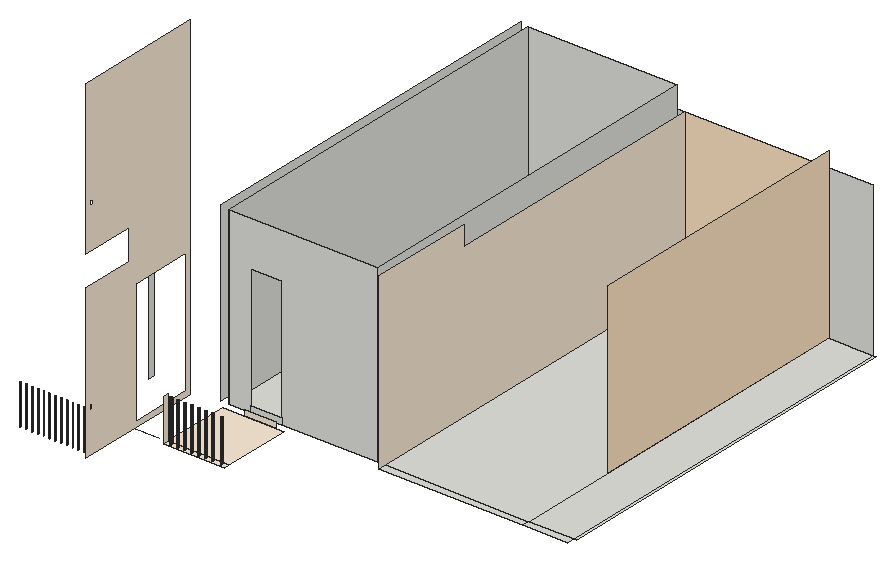
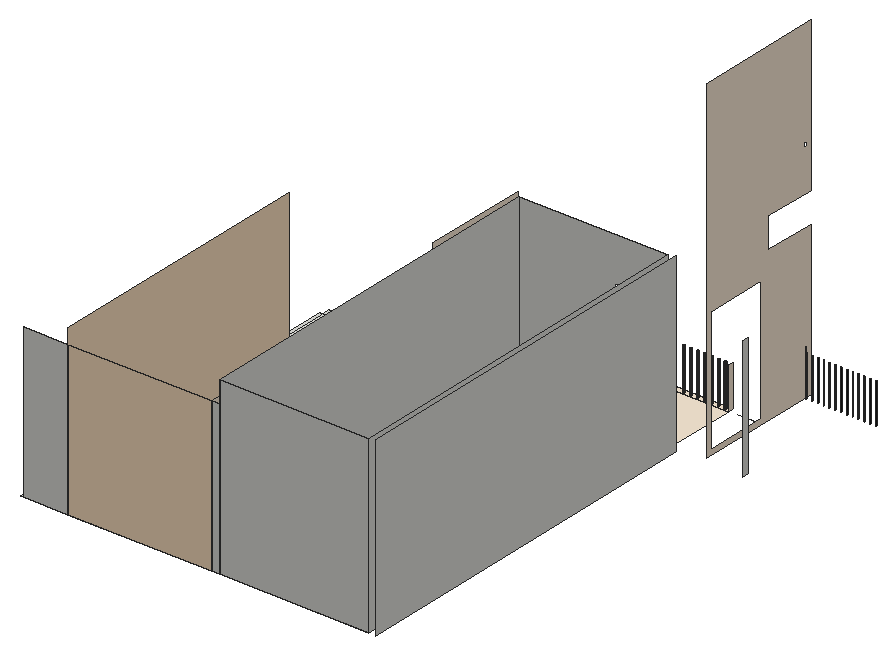
# SketchUp Ruby script. Lengths in inches.
U = 1.inch
M = Sketchup.active_model
def pt(a) = Geom::Point3d.new(a.map { |v| v * U })
def face(e, loops, mat)
  f = e.add_face(loops[0].map { |a| pt(a) })
  loops[1..].each { |l| e.add_face(l.map { |a| pt(a) }).erase! }
  f.material = f.back_material = mat if mat
  f
end
# faces: each face lists its corners as indices into pts; further lists are holes
def faces(e, pts, list, mat = nil) = list.each { |f| face(e, (f[0].is_a?(Array) ? f : [f]).map { |l| l.map { |i| pts[i] } }, mat) }
# xy, xz, yz: faces in a plane at the given z, y or x. An outline is a flat list of corners, or four numbers for a rectangle; further outlines are holes
def ring(l) = l.size == 4 ? [[l[0], l[1]], [l[2], l[1]], [l[2], l[3]], [l[0], l[3]]] : l.each_slice(2).to_a
def flat(e, list, mat, &to3) = list.each { |f| face(e, (f[0].is_a?(Array) ? f : [f]).map { |l| ring(l).map { |u, v| to3.(u, v) } }, mat) }
def xy(e, z, list, mat = nil) = flat(e, list, mat) { |x, y| [x, y, z] }
def xz(e, y, list, mat = nil) = flat(e, list, mat) { |x, z| [x, y, z] }
def yz(e, x, list, mat = nil) = flat(e, list, mat) { |y, z| [x, y, z] }
def lines(e, pts, list) = list.each { |a, b| e.add_line(pt(pts[a]), pt(pts[b])) }
# prism: a flat outline (further loops are holes) pulled along v
def prism(e, loops, v, mat = nil)
  f = face(e, loops, mat); d = Geom::Vector3d.new(v.map { |x| x * U })
  f.pushpull(f.normal.samedirection?(d) ? d.length : -d.length)
end
def box(e, o, s, mat = nil) = prism(e, [[o, [o[0] + s[0], o[1], o[2]], [o[0] + s[0], o[1] + s[1], o[2]], [o[0], o[1] + s[1], o[2]]]], [0, 0, s[2]], mat)
def at(x, y, z, deg = 0) = Geom::Transformation.translation(pt([x, y, z])) * Geom::Transformation.rotation(ORIGIN, Z_AXIS, deg.degrees)
def axes(o, x, y, z) = Geom::Transformation.new([*x, 0, *y, 0, *z, 0, *pt(o).to_a, 1])
def part(name) = M.definitions.add(name)
# library, detail: a bought-in or finely detailed component or shape, given as its bounding box
def library(name, o, s) = part(name).tap { |d| box(d.entities, o, s) }
def detail(e, o, s) = box(e.add_group.entities, o, s)
def put(e, d, t, mat = nil) = e.add_instance(d, t).tap { |i| i.material = mat if mat }
def group(e, t, mat = nil) = e.add_group.tap { |g| g.transformation = t; g.material = mat if mat }.entities
root = M.entities
M.materials.add("[0012_Bisque]").color = [255, 228, 196]
M.materials.add("[0028_AntiqueWhite]").color = [250, 235, 215]
M.materials.add("[Color M08]").color = [30, 30, 30]
xy(root,177,[[355.625,292.4375,468.75,298.4375],[468.75,292.4375,503.75,298.4375],[232.3125,298.4375,349.625,592.9375],[355.625,298.4375,468.75,592.9375],[468.75,298.4375,503.75,592.9375],
  [503.75,298.4375,506.4375,592.9375]])
xy(root,177,[[[232.3125,234.5,280.54,238.33],[242.01,235.93,241.83,235.95,241.66,236.02,241.52,236.12,241.41,236.26,241.34,236.43,241.31,236.61,241.33,236.78,241.39,236.95,241.5,237.09,241.64,237.21,241.81,237.28,241.98,237.31,242.16,237.29,242.33,237.22,242.47,237.11,242.58,236.97,242.66,236.81,242.68,236.63,242.66,236.45,242.6,236.29,242.49,236.14,242.35,236.03,242.1875,235.96],[247.45,235.93,247.27,235.95,247.1,236.02,246.96,236.12,246.84,236.26,246.77,236.43,246.75,236.61,246.77,236.78,246.83,236.95,246.9375,237.09,247.08,237.21,247.24,237.28,247.42,237.31,247.6,237.29,247.77,237.22,247.91,237.11,248.02,236.97,248.09,236.81,248.12,236.63,248.1,236.45,248.04,236.29,247.93,236.14,247.79,236.03,247.625,235.96],[252.88,235.93,252.71,235.95,252.54,236.02,252.39,236.12,252.28,236.26,252.21,236.43,252.18,236.61,252.2,236.78,252.27,236.95,252.375,237.09,252.52,237.21,252.68,237.28,252.86,237.31,253.04,237.29,253.2,237.22,253.35,237.11,253.46,236.97,253.53,236.81,253.56,236.63,253.54,236.45,253.47,236.29,253.37,236.14,253.23,236.03,253.0625,235.96],[258.32,235.93,258.14,235.95,257.98,236.02,257.83,236.12,257.72,236.26,257.65,236.43,257.62,236.61,257.64,236.78,257.71,236.95,257.8125,237.09,257.95,237.21,258.12,237.28,258.3,237.31,258.47,237.29,258.64,237.22,258.79,237.11,258.9,236.97,258.97,236.81,259,236.63,258.98,236.45,258.91,236.29,258.8,236.14,258.66,236.03,258.5,235.96],[263.76,235.93,263.58,235.95,263.41,236.02,263.27,236.12,263.16,236.26,263.09,236.43,263.06,236.61,263.08,236.78,263.14,236.95,263.25,237.09,263.39,237.21,263.56,237.28,263.73,237.31,263.91,237.29,264.08,237.22,264.22,237.11,264.33,236.97,264.41,236.81,264.43,236.63,264.41,236.45,264.35,236.29,264.24,236.14,264.1,236.03,263.9375,235.96],[269.26,235.93,269.08,235.95,268.91,236.02,268.77,236.12,268.66,236.26,268.59,236.43,268.56,236.61,268.58,236.78,268.64,236.95,268.75,237.09,268.89,237.21,269.06,237.28,269.23,237.31,269.41,237.29,269.58,237.22,269.72,237.11,269.83,236.97,269.91,236.81,269.93,236.63,269.91,236.45,269.85,236.29,269.74,236.14,269.6,236.03,269.4375,235.96],[276.2,235.93,276.02,235.95,275.85,236.02,275.71,236.12,275.59,236.26,275.52,236.43,275.5,236.61,275.52,236.78,275.58,236.95,275.6875,237.09,275.83,237.21,275.99,237.28,276.17,237.31,276.35,237.29,276.52,237.22,276.66,237.11,276.77,236.97,276.84,236.81,276.87,236.63,276.85,236.45,276.79,236.29,276.68,236.14,276.54,236.03,276.375,235.96],[236.57,235.93,236.39,235.95,236.23,236.02,236.08,236.12,235.97,236.26,235.9,236.43,235.87,236.61,235.89,236.78,235.96,236.95,236.0625,237.09,236.2,237.21,236.37,237.28,236.55,237.31,236.72,237.29,236.89,237.22,237.04,237.11,237.15,236.97,237.22,236.81,237.25,236.63,237.23,236.45,237.16,236.29,237.05,236.14,236.91,236.03,236.75,235.96]],[232.3125,238.33,280.54,292.4375]],"[0028_AntiqueWhite]")
xy(root,177,[[236.57,235.93,236.39,235.95,236.23,236.02,236.08,236.12,235.97,236.26,235.9,236.43,235.87,236.61,235.89,236.78,235.96,236.95,236.0625,237.09,236.2,237.21,236.37,237.28,236.55,237.31,236.72,237.29,236.89,237.22,237.04,237.11,237.15,236.97,237.22,236.81,237.25,236.63,237.23,236.45,237.16,236.29,237.05,236.14,236.91,236.03,236.75,235.96],[242.01,235.93,241.83,235.95,241.66,236.02,241.52,236.12,241.41,236.26,241.34,236.43,241.31,236.61,241.33,236.78,241.39,236.95,241.5,237.09,241.64,237.21,241.81,237.28,241.98,237.31,242.16,237.29,242.33,237.22,242.47,237.11,242.58,236.97,242.66,236.81,242.68,236.63,242.66,236.45,242.6,236.29,242.49,236.14,242.35,236.03,242.1875,235.96],[247.45,235.93,247.27,235.95,247.1,236.02,246.96,236.12,246.84,236.26,246.77,236.43,246.75,236.61,246.77,236.78,246.83,236.95,246.9375,237.09,247.08,237.21,247.24,237.28,247.42,237.31,247.6,237.29,247.77,237.22,247.91,237.11,248.02,236.97,248.09,236.81,248.12,236.63,248.1,236.45,248.04,236.29,247.93,236.14,247.79,236.03,247.625,235.96],[252.88,235.93,252.71,235.95,252.54,236.02,252.39,236.12,252.28,236.26,252.21,236.43,252.18,236.61,252.2,236.78,252.27,236.95,252.375,237.09,252.52,237.21,252.68,237.28,252.86,237.31,253.04,237.29,253.2,237.22,253.35,237.11,253.46,236.97,253.53,236.81,253.56,236.63,253.54,236.45,253.47,236.29,253.37,236.14,253.23,236.03,253.0625,235.96],[258.32,235.93,258.14,235.95,257.98,236.02,257.83,236.12,257.72,236.26,257.65,236.43,257.62,236.61,257.64,236.78,257.71,236.95,257.8125,237.09,257.95,237.21,258.12,237.28,258.3,237.31,258.47,237.29,258.64,237.22,258.79,237.11,258.9,236.97,258.97,236.81,259,236.63,258.98,236.45,258.91,236.29,258.8,236.14,258.66,236.03,258.5,235.96],
  [263.76,235.93,263.58,235.95,263.41,236.02,263.27,236.12,263.16,236.26,263.09,236.43,263.06,236.61,263.08,236.78,263.14,236.95,263.25,237.09,263.39,237.21,263.56,237.28,263.73,237.31,263.91,237.29,264.08,237.22,264.22,237.11,264.33,236.97,264.41,236.81,264.43,236.63,264.41,236.45,264.35,236.29,264.24,236.14,264.1,236.03,263.9375,235.96],[269.26,235.93,269.08,235.95,268.91,236.02,268.77,236.12,268.66,236.26,268.59,236.43,268.56,236.61,268.58,236.78,268.64,236.95,268.75,237.09,268.89,237.21,269.06,237.28,269.23,237.31,269.41,237.29,269.58,237.22,269.72,237.11,269.83,236.97,269.91,236.81,269.93,236.63,269.91,236.45,269.85,236.29,269.74,236.14,269.6,236.03,269.4375,235.96],[276.2,235.93,276.02,235.95,275.85,236.02,275.71,236.12,275.59,236.26,275.52,236.43,275.5,236.61,275.52,236.78,275.58,236.95,275.6875,237.09,275.83,237.21,275.99,237.28,276.17,237.31,276.35,237.29,276.52,237.22,276.66,237.11,276.77,236.97,276.84,236.81,276.87,236.63,276.85,236.45,276.79,236.29,276.68,236.14,276.54,236.03,276.375,235.96]],"[Color M08]")
xz(root,195.79,[[150.6,177,150.75,208.66],[155.17,177,155.3125,208.66],[159.73,177,159.875,208.66],[164.29,177,164.4375,208.66],[168.85,177,169,208.66],
  [173.42,177,173.5625,208.625],[177.98,177,178.125,208.66],[182.54,177,182.6875,208.66],[187.1,177,187.25,208.66],[191.67,177,191.8125,208.66],
  [196.23,177,196.375,208.66],[200.79,177,200.9375,208.66],[205.35,177,205.5,208.9375]],"[Color M08]")
xz(root,292.4375,[[249.93,177,274.3,181.75]],"[0028_AntiqueWhite]")
xz(root,298.4375,[[232.3125,177,232.3125,313.625,349.625,313.625,349.625,177,274.3,177,274.3,278.54,249.93,278.54,249.93,177],[249.93,177,274.3,181.75]])
xz(root,592.9375,[[232.3125,177,349.625,313.625],[349.625,177,355.625,297],[468.75,177,503.75,297]])
xz(root,592.9375,[[355.625,177,468.75,297]],"[0012_Bisque]")
yz(root,206.5625,[[[190.5,177,190.5,297,231.9375,297,231.9375,321,190.5,321,190.5,441,292.44,441,292.44,177],[238.8,181.1,288.24,278.41],[193.58,208.66,196.4375,208.66,196.4375,213,193.51,213],[193.51,353.72,196.625,357]]],"[0028_AntiqueWhite]")
yz(root,226.3125,[[298.4375,177,592.9375,315]])
yz(root,232.3125,[[298.4375,177,592.9375,313.625]])
yz(root,232.3125,[[234.5,177,238.33,209.97]],"[0028_AntiqueWhite]")
yz(root,349.625,[[298.4375,177,592.9375,313.625]])
yz(root,355.625,[[292.4375,177,592.9375,177,592.9375,297,375.81,297,375.81,312.75,292.4375,312.75]],"[0028_AntiqueWhite]")
yz(root,468.75,[[376.0625,177,592.9375,309]],"[0012_Bisque]")
p = [[164.71,195.68,177],[164.58,195.75,177],[164.58,195.75,208.66],[164.71,195.68,208.66],[169.27,195.68,177],[169.14,195.75,177],
  [169.14,195.75,208.66],[169.27,195.68,208.66],[173.83,195.68,177],[173.7,195.75,177],[173.7,195.75,208.625],[173.83,195.68,208.625],
  [178.39,195.68,177],[178.27,195.75,177],[178.27,195.75,208.66],[178.39,195.68,208.66],[182.96,195.68,177],[182.83,195.75,177],
  [182.83,195.75,208.66],[182.96,195.68,208.66],[187.52,195.68,177],[187.39,195.75,177],[187.39,195.75,208.66],[187.52,195.68,208.66],
  [192.08,195.68,177],[191.95,195.75,177],[191.95,195.75,208.66],[192.08,195.68,208.66],[196.64,195.68,177],[196.52,195.75,177],
  [196.52,195.75,208.66],[196.64,195.68,208.66],[201.21,195.68,177],[201.08,195.75,177],[201.08,195.75,208.66],[201.21,195.68,208.66],
  [205.77,195.68,177],[205.64,195.75,177],[205.64,195.75,208.9375],[205.77,195.68,208.9375],[150.6,195.79,177],[150.46,195.75,177],
  [150.46,195.75,208.66],[150.6,195.79,208.66],[150.89,195.75,177],[150.75,195.79,177],[150.75,195.79,208.66],[150.89,195.75,208.66],
  [155.17,195.79,177],[155.02,195.75,177],[155.02,195.75,208.66],[155.17,195.79,208.66],[155.45,195.75,177],[155.3125,195.79,177],
  [155.3125,195.79,208.66],[155.45,195.75,208.66],[159.73,195.79,177],[159.59,195.75,177],[159.59,195.75,208.66],[159.73,195.79,208.66],
  [160.02,195.75,177],[159.875,195.79,177],[159.875,195.79,208.66],[160.02,195.75,208.66],[164.29,195.79,177],[164.15,195.75,177],
  [164.15,195.75,208.66],[164.29,195.79,208.66],[164.4375,195.79,177],[164.4375,195.79,208.66],[168.85,195.79,177],[168.71,195.75,177],
  [168.71,195.75,208.66],[168.85,195.79,208.66],[169,195.79,177],[169,195.79,208.66],[173.42,195.79,177],[173.27,195.75,177],
  [173.27,195.75,208.625],[173.42,195.79,208.625],[173.5625,195.79,177],[173.5625,195.79,208.625],[177.98,195.79,177],[177.84,195.75,177],
  [177.84,195.75,208.66],[177.98,195.79,208.66],[178.125,195.79,177],[178.125,195.79,208.66],[182.54,195.79,177],[182.4,195.75,177],
  [182.4,195.75,208.66],[182.54,195.79,208.66],[182.6875,195.79,177],[182.6875,195.79,208.66],[187.1,195.79,177],[186.96,195.75,177],
  [186.96,195.75,208.66],[187.1,195.79,208.66],[187.25,195.79,177],[187.25,195.79,208.66],[191.67,195.79,177],[191.52,195.75,177],
  [191.52,195.75,208.66],[191.67,195.79,208.66],[191.8125,195.79,177],[191.8125,195.79,208.66],[196.23,195.79,177],[196.09,195.75,177],
  [196.09,195.75,208.66],[196.23,195.79,208.66],[196.375,195.79,177],[196.375,195.79,208.66],[200.79,195.79,177],[200.65,195.75,177],
  [200.65,195.75,208.66],[200.79,195.79,208.66],[200.9375,195.79,177],[200.9375,195.79,208.66],[205.35,195.79,177],[205.21,195.75,177],
  [205.21,195.75,208.9375],[205.35,195.79,208.9375],[205.5,195.79,177],[205.5,195.79,208.9375],[236.39,235.95,177],[236.57,235.93,177],
  [236.57,235.93,209.97],[236.39,235.95,209.97],[236.75,235.96,177],[236.75,235.96,209.97],[241.83,235.95,177],[242.01,235.93,177],
  [242.01,235.93,209.97],[241.83,235.95,209.97],[242.1875,235.96,177],[242.1875,235.96,209.97],[247.27,235.95,177],[247.45,235.93,177],
  [247.45,235.93,209.97],[247.27,235.95,209.97],[247.625,235.96,177],[247.625,235.96,209.97],[252.71,235.95,177],[252.88,235.93,177],
  [252.88,235.93,209.97],[252.71,235.95,209.97],[253.0625,235.96,177],[253.0625,235.96,209.97],[258.14,235.95,177],[258.32,235.93,177],
  [258.32,235.93,209.97],[258.14,235.95,209.97],[258.5,235.96,177],[258.5,235.96,209.97],[263.58,235.95,177],[263.76,235.93,177],
  [263.76,235.93,209.97],[263.58,235.95,209.97],[263.9375,235.96,177],[263.9375,235.96,209.97],[269.08,235.95,177],[269.26,235.93,177],
  [269.26,235.93,209.97],[269.08,235.95,209.97],[269.4375,235.96,177],[269.4375,235.96,209.97],[276.02,235.95,177],[276.2,235.93,177],
  [276.2,235.93,209.97],[276.02,235.95,209.97],[276.375,235.96,177],[276.375,235.96,209.97],[236.08,236.12,177],[236.23,236.02,177],
  [236.23,236.02,209.97],[236.08,236.12,209.97],[236.91,236.03,177],[236.91,236.03,209.97],[237.05,236.14,177],[237.05,236.14,209.97],
  [241.52,236.12,177],[241.66,236.02,177],[241.66,236.02,209.97],[241.52,236.12,209.97],[242.35,236.03,177],[242.35,236.03,209.97],
  [242.49,236.14,177],[242.49,236.14,209.97],[246.96,236.12,177],[247.1,236.02,177],[247.1,236.02,209.97],[246.96,236.12,209.97],
  [247.79,236.03,177],[247.79,236.03,209.97],[247.93,236.14,177],[247.93,236.14,209.97],[252.39,236.12,177],[252.54,236.02,177],
  [252.54,236.02,209.97],[252.39,236.12,209.97],[253.23,236.03,177],[253.23,236.03,209.97],[253.37,236.14,177],[253.37,236.14,209.97],
  [257.83,236.12,177],[257.98,236.02,177],[257.98,236.02,209.97],[257.83,236.12,209.97],[258.66,236.03,177],[258.66,236.03,209.97],
  [258.8,236.14,177],[258.8,236.14,209.97],[263.27,236.12,177],[263.41,236.02,177],[263.41,236.02,209.97],[263.27,236.12,209.97],
  [264.1,236.03,177],[264.1,236.03,209.97],[264.24,236.14,177],[264.24,236.14,209.97],[268.77,236.12,177],[268.91,236.02,177],
  [268.91,236.02,209.97],[268.77,236.12,209.97],[269.6,236.03,177],[269.6,236.03,209.97],[269.74,236.14,177],[269.74,236.14,209.97],
  [275.71,236.12,177],[275.85,236.02,177],[275.85,236.02,209.97],[275.71,236.12,209.97],[276.54,236.03,177],[276.54,236.03,209.97],
  [276.68,236.14,177],[276.68,236.14,209.97],[235.97,236.26,177],[235.97,236.26,209.97],[237.16,236.29,177],[237.16,236.29,209.97],
  [241.41,236.26,177],[241.41,236.26,209.97],[242.6,236.29,177],[242.6,236.29,209.97],[246.84,236.26,177],[246.84,236.26,209.97],
  [248.04,236.29,177],[248.04,236.29,209.97],[252.28,236.26,177],[252.28,236.26,209.97],[253.47,236.29,177],[253.47,236.29,209.97],
  [257.72,236.26,177],[257.72,236.26,209.97],[258.91,236.29,177],[258.91,236.29,209.97],[263.16,236.26,177],[263.16,236.26,209.97],
  [264.35,236.29,177],[264.35,236.29,209.97],[268.66,236.26,177],[268.66,236.26,209.97],[269.85,236.29,177],[269.85,236.29,209.97],
  [275.59,236.26,177],[275.59,236.26,209.97],[276.79,236.29,177],[276.79,236.29,209.97],[235.9,236.43,177],[235.9,236.43,209.97],
  [237.23,236.45,177],[237.23,236.45,209.97],[241.34,236.43,177],[241.34,236.43,209.97],[242.66,236.45,177],[242.66,236.45,209.97],
  [246.77,236.43,177],[246.77,236.43,209.97],[248.1,236.45,177],[248.1,236.45,209.97],[252.21,236.43,177],[252.21,236.43,209.97],
  [253.54,236.45,177],[253.54,236.45,209.97],[257.65,236.43,177],[257.65,236.43,209.97],[258.98,236.45,177],[258.98,236.45,209.97],
  [263.09,236.43,177],[263.09,236.43,209.97],[264.41,236.45,177],[264.41,236.45,209.97],[268.59,236.43,177],[268.59,236.43,209.97],
  [269.91,236.45,177],[269.91,236.45,209.97],[275.52,236.43,177],[275.52,236.43,209.97],[276.85,236.45,177],[276.85,236.45,209.97],
  [235.87,236.61,177],[235.87,236.61,209.97],[241.31,236.61,177],[241.31,236.61,209.97],[246.75,236.61,177],[246.75,236.61,209.97],
  [252.18,236.61,177],[252.18,236.61,209.97],[257.62,236.61,177],[257.62,236.61,209.97],[263.06,236.61,177],[263.06,236.61,209.97],
  [268.56,236.61,177],[268.56,236.61,209.97],[275.5,236.61,177],[275.5,236.61,209.97],[237.25,236.63,177],[237.25,236.63,209.97],
  [242.68,236.63,177],[242.68,236.63,209.97],[248.12,236.63,177],[248.12,236.63,209.97],[253.56,236.63,177],[253.56,236.63,209.97],
  [259,236.63,177],[259,236.63,209.97],[264.43,236.63,177],[264.43,236.63,209.97],[269.93,236.63,177],[269.93,236.63,209.97],
  [276.87,236.63,177],[276.87,236.63,209.97],[235.89,236.78,177],[235.89,236.78,209.97],[237.22,236.81,177],[237.22,236.81,209.97],
  [241.33,236.78,177],[241.33,236.78,209.97],[242.66,236.81,177],[242.66,236.81,209.97],[246.77,236.78,177],[246.77,236.78,209.97],
  [248.09,236.81,177],[248.09,236.81,209.97],[252.2,236.78,177],[252.2,236.78,209.97],[253.53,236.81,177],[253.53,236.81,209.97],
  [257.64,236.78,177],[257.64,236.78,209.97],[258.97,236.81,177],[258.97,236.81,209.97],[263.08,236.78,177],[263.08,236.78,209.97],
  [264.41,236.81,177],[264.41,236.81,209.97],[268.58,236.78,177],[268.58,236.78,209.97],[269.91,236.81,177],[269.91,236.81,209.97],
  [275.52,236.78,177],[275.52,236.78,209.97],[276.84,236.81,177],[276.84,236.81,209.97],[235.96,236.95,177],[235.96,236.95,209.97],
  [237.15,236.97,177],[237.15,236.97,209.97],[241.39,236.95,177],[241.39,236.95,209.97],[242.58,236.97,177],[242.58,236.97,209.97],
  [246.83,236.95,177],[246.83,236.95,209.97],[248.02,236.97,177],[248.02,236.97,209.97],[252.27,236.95,177],[252.27,236.95,209.97],
  [253.46,236.97,177],[253.46,236.97,209.97],[257.71,236.95,177],[257.71,236.95,209.97],[258.9,236.97,177],[258.9,236.97,209.97],
  [263.14,236.95,177],[263.14,236.95,209.97],[264.33,236.97,177],[264.33,236.97,209.97],[268.64,236.95,177],[268.64,236.95,209.97],
  [269.83,236.97,177],[269.83,236.97,209.97],[275.58,236.95,177],[275.58,236.95,209.97],[276.77,236.97,177],[276.77,236.97,209.97],
  [236.0625,237.09,177],[236.0625,237.09,209.97],[237.04,237.11,177],[237.04,237.11,209.97],[241.5,237.09,177],[241.5,237.09,209.97],
  [242.47,237.11,177],[242.47,237.11,209.97],[246.9375,237.09,177],[246.9375,237.09,209.97],[247.91,237.11,177],[247.91,237.11,209.97],
  [252.375,237.09,177],[252.375,237.09,209.97],[253.35,237.11,177],[253.35,237.11,209.97],[257.8125,237.09,177],[257.8125,237.09,209.97],
  [258.79,237.11,177],[258.79,237.11,209.97],[263.25,237.09,177],[263.25,237.09,209.97],[264.22,237.11,177],[264.22,237.11,209.97],
  [268.75,237.09,177],[268.75,237.09,209.97],[269.72,237.11,177],[269.72,237.11,209.97],[275.6875,237.09,177],[275.6875,237.09,209.97],
  [276.66,237.11,177],[276.66,237.11,209.97],[236.2,237.21,177],[236.2,237.21,209.97],[236.89,237.22,177],[236.89,237.22,209.97],
  [241.64,237.21,177],[241.64,237.21,209.97],[242.33,237.22,177],[242.33,237.22,209.97],[247.08,237.21,177],[247.08,237.21,209.97],
  [247.77,237.22,177],[247.77,237.22,209.97],[252.52,237.21,177],[252.52,237.21,209.97],[253.2,237.22,177],[253.2,237.22,209.97],
  [257.95,237.21,177],[257.95,237.21,209.97],[258.64,237.22,177],[258.64,237.22,209.97],[263.39,237.21,177],[263.39,237.21,209.97],
  [264.08,237.22,177],[264.08,237.22,209.97],[268.89,237.21,177],[268.89,237.21,209.97],[269.58,237.22,177],[269.58,237.22,209.97],
  [275.83,237.21,177],[275.83,237.21,209.97],[276.52,237.22,177],[276.52,237.22,209.97],[236.37,237.28,177],[236.37,237.28,209.97],
  [236.72,237.29,177],[236.72,237.29,209.97],[241.81,237.28,177],[241.81,237.28,209.97],[242.16,237.29,177],[242.16,237.29,209.97],
  [247.24,237.28,177],[247.24,237.28,209.97],[247.6,237.29,177],[247.6,237.29,209.97],[252.68,237.28,177],[252.68,237.28,209.97],
  [253.04,237.29,177],[253.04,237.29,209.97],[258.12,237.28,177],[258.12,237.28,209.97],[258.47,237.29,177],[258.47,237.29,209.97],
  [263.56,237.28,177],[263.56,237.28,209.97],[263.91,237.29,177],[263.91,237.29,209.97],[269.06,237.28,177],[269.06,237.28,209.97],
  [269.41,237.29,177],[269.41,237.29,209.97],[275.99,237.28,177],[275.99,237.28,209.97],[276.35,237.29,177],[276.35,237.29,209.97],
  [236.55,237.31,177],[236.55,237.31,209.97],[241.98,237.31,177],[241.98,237.31,209.97],[247.42,237.31,177],[247.42,237.31,209.97],
  [252.86,237.31,177],[252.86,237.31,209.97],[258.3,237.31,177],[258.3,237.31,209.97],[263.73,237.31,177],[263.73,237.31,209.97],
  [269.23,237.31,177],[269.23,237.31,209.97],[276.17,237.31,177],[276.17,237.31,209.97],[174.56,292.48,177],[174.56,292.48,272.875],
  [174.5625,296.73,272.875],[174.5625,296.73,177],[226.3125,237.9375,177],[206.5625,237.9375,177]]
faces(root,p,[[0,1,2,3],[4,5,6,7],[8,9,10,11],[12,13,14,15],[16,17,18,19],[20,21,22,23],[24,25,26,27],[28,29,30,31],
  [32,33,34,35],[36,37,38,39],[40,41,42,43],[44,45,46,47],[48,49,50,51],[52,53,54,55],[56,57,58,59],[60,61,62,63],
  [64,65,66,67],[1,68,69,2],[70,71,72,73],[5,74,75,6],[76,77,78,79],[9,80,81,10],[82,83,84,85],[13,86,87,14],
  [88,89,90,91],[17,92,93,18],[94,95,96,97],[21,98,99,22],[100,101,102,103],[25,104,105,26],[106,107,108,109],[29,110,111,30],
  [112,113,114,115],[33,116,117,34],[118,119,120,121],[37,122,123,38],[124,125,126,127],[125,128,129,126],[130,131,132,133],[131,134,135,132],
  [136,137,138,139],[137,140,141,138],[142,143,144,145],[143,146,147,144],[148,149,150,151],[149,152,153,150],[154,155,156,157],[155,158,159,156],
  [160,161,162,163],[161,164,165,162],[166,167,168,169],[167,170,171,168],[172,173,174,175],[173,124,127,174],[128,176,177,129],[176,178,179,177],
  [180,181,182,183],[181,130,133,182],[134,184,185,135],[184,186,187,185],[188,189,190,191],[189,136,139,190],[140,192,193,141],[192,194,195,193],
  [196,197,198,199],[197,142,145,198],[146,200,201,147],[200,202,203,201],[204,205,206,207],[205,148,151,206],[152,208,209,153],[208,210,211,209],
  [212,213,214,215],[213,154,157,214],[158,216,217,159],[216,218,219,217],[220,221,222,223],[221,160,163,222],[164,224,225,165],[224,226,227,225],
  [228,229,230,231],[229,166,169,230],[170,232,233,171],[232,234,235,233],[236,172,175,237],[178,238,239,179],[240,180,183,241],[186,242,243,187],
  [244,188,191,245],[194,246,247,195],[248,196,199,249],[202,250,251,203],[252,204,207,253],[210,254,255,211],[256,212,215,257],[218,258,259,219],
  [260,220,223,261],[226,262,263,227],[264,228,231,265],[234,266,267,235],[268,236,237,269],[238,270,271,239],[272,240,241,273],[242,274,275,243],
  [276,244,245,277],[246,278,279,247],[280,248,249,281],[250,282,283,251],[284,252,253,285],[254,286,287,255],[288,256,257,289],[258,290,291,259],
  [292,260,261,293],[262,294,295,263],[296,264,265,297],[266,298,299,267],[300,268,269,301],[302,272,273,303],[304,276,277,305],[306,280,281,307],
  [308,284,285,309],[310,288,289,311],[312,292,293,313],[314,296,297,315],[270,316,317,271],[274,318,319,275],[278,320,321,279],[282,322,323,283],
  [286,324,325,287],[290,326,327,291],[294,328,329,295],[298,330,331,299],[332,300,301,333],[316,334,335,317],[336,302,303,337],[318,338,339,319],
  [340,304,305,341],[320,342,343,321],[344,306,307,345],[322,346,347,323],[348,308,309,349],[324,350,351,325],[352,310,311,353],[326,354,355,327],
  [356,312,313,357],[328,358,359,329],[360,314,315,361],[330,362,363,331],[364,332,333,365],[334,366,367,335],[368,336,337,369],[338,370,371,339],
  [372,340,341,373],[342,374,375,343],[376,344,345,377],[346,378,379,347],[380,348,349,381],[350,382,383,351],[384,352,353,385],[354,386,387,355],
  [388,356,357,389],[358,390,391,359],[392,360,361,393],[362,394,395,363],[396,364,365,397],[366,398,399,367],[400,368,369,401],[370,402,403,371],
  [404,372,373,405],[374,406,407,375],[408,376,377,409],[378,410,411,379],[412,380,381,413],[382,414,415,383],[416,384,385,417],[386,418,419,387],
  [420,388,389,421],[390,422,423,391],[424,392,393,425],[394,426,427,395],[428,396,397,429],[398,430,431,399],[432,400,401,433],[402,434,435,403],
  [436,404,405,437],[406,438,439,407],[440,408,409,441],[410,442,443,411],[444,412,413,445],[414,446,447,415],[448,416,417,449],[418,450,451,419],
  [452,420,421,453],[422,454,455,423],[456,424,425,457],[426,458,459,427],[460,428,429,461],[430,462,463,431],[464,432,433,465],[434,466,467,435],
  [468,436,437,469],[438,470,471,439],[472,440,441,473],[442,474,475,443],[476,444,445,477],[446,478,479,447],[480,448,449,481],[450,482,483,451],
  [484,452,453,485],[454,486,487,455],[488,456,457,489],[458,490,491,459],[492,460,461,493],[462,492,493,463],[494,464,465,495],[466,494,495,467],
  [496,468,469,497],[470,496,497,471],[498,472,473,499],[474,498,499,475],[500,476,477,501],[478,500,501,479],[502,480,481,503],[482,502,503,483],
  [504,484,485,505],[486,504,505,487],[506,488,489,507],[490,506,507,491]],"[Color M08]")
faces(root,p,[[508,509,510,511]])
lines(root,p,[[512,513]])
